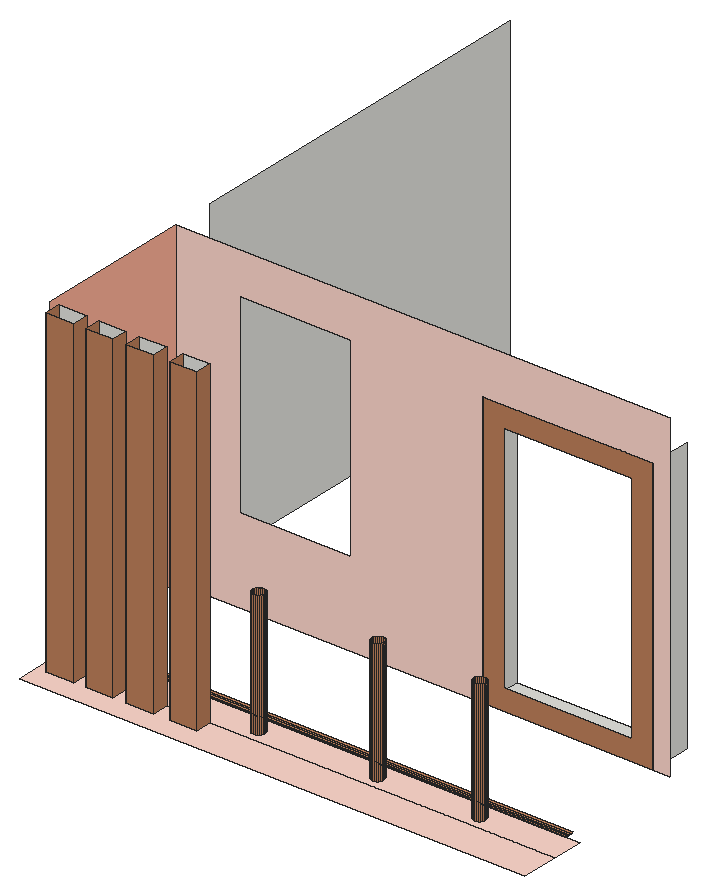
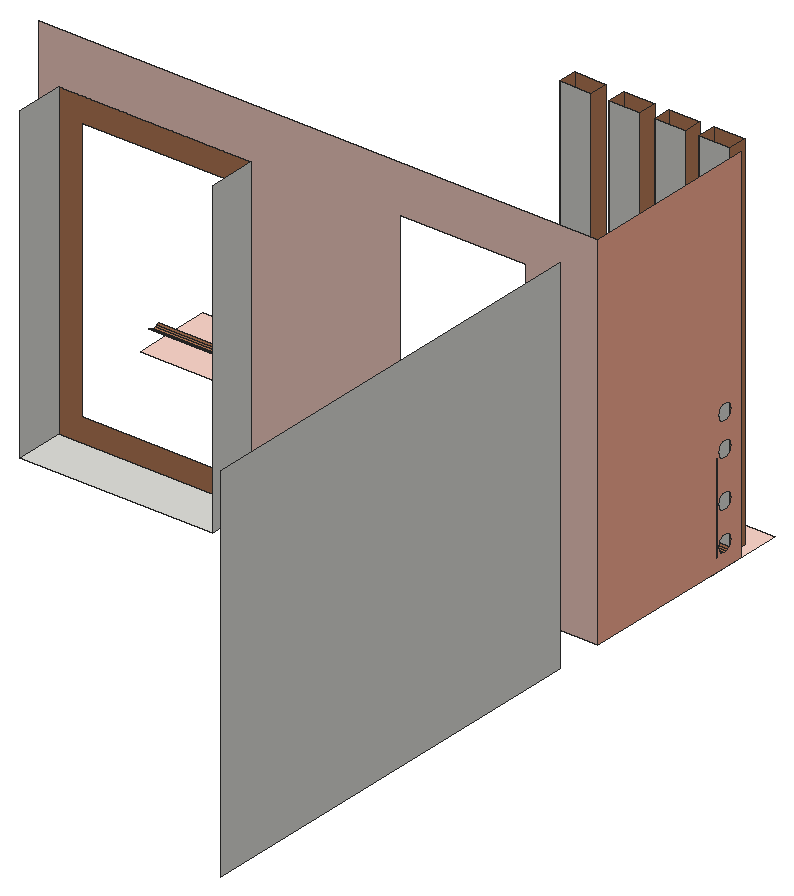
# SketchUp Ruby script. Lengths in inches.
U = 1.inch
M = Sketchup.active_model
def pt(a) = Geom::Point3d.new(a.map { |v| v * U })
def face(e, loops, mat)
  f = e.add_face(loops[0].map { |a| pt(a) })
  loops[1..].each { |l| e.add_face(l.map { |a| pt(a) }).erase! }
  f.material = f.back_material = mat if mat
  f
end
# faces: each face lists its corners as indices into pts; further lists are holes
def faces(e, pts, list, mat = nil) = list.each { |f| face(e, (f[0].is_a?(Array) ? f : [f]).map { |l| l.map { |i| pts[i] } }, mat) }
# xy, xz, yz: faces in a plane at the given z, y or x. An outline is a flat list of corners, or four numbers for a rectangle; further outlines are holes
def ring(l) = l.size == 4 ? [[l[0], l[1]], [l[2], l[1]], [l[2], l[3]], [l[0], l[3]]] : l.each_slice(2).to_a
def flat(e, list, mat, &to3) = list.each { |f| face(e, (f[0].is_a?(Array) ? f : [f]).map { |l| ring(l).map { |u, v| to3.(u, v) } }, mat) }
def xy(e, z, list, mat = nil) = flat(e, list, mat) { |x, y| [x, y, z] }
def xz(e, y, list, mat = nil) = flat(e, list, mat) { |x, z| [x, y, z] }
def yz(e, x, list, mat = nil) = flat(e, list, mat) { |y, z| [x, y, z] }
def lines(e, pts, list) = list.each { |a, b| e.add_line(pt(pts[a]), pt(pts[b])) }
# prism: a flat outline (further loops are holes) pulled along v
def prism(e, loops, v, mat = nil)
  f = face(e, loops, mat); d = Geom::Vector3d.new(v.map { |x| x * U })
  f.pushpull(f.normal.samedirection?(d) ? d.length : -d.length)
end
def box(e, o, s, mat = nil) = prism(e, [[o, [o[0] + s[0], o[1], o[2]], [o[0] + s[0], o[1] + s[1], o[2]], [o[0], o[1] + s[1], o[2]]]], [0, 0, s[2]], mat)
def at(x, y, z, deg = 0) = Geom::Transformation.translation(pt([x, y, z])) * Geom::Transformation.rotation(ORIGIN, Z_AXIS, deg.degrees)
def axes(o, x, y, z) = Geom::Transformation.new([*x, 0, *y, 0, *z, 0, *pt(o).to_a, 1])
def part(name) = M.definitions.add(name)
# library, detail: a bought-in or finely detailed component or shape, given as its bounding box
def library(name, o, s) = part(name).tap { |d| box(d.entities, o, s) }
def detail(e, o, s) = box(e.add_group.entities, o, s)
def put(e, d, t, mat = nil) = e.add_instance(d, t).tap { |i| i.material = mat if mat }
def group(e, t, mat = nil) = e.add_group.tap { |g| g.transformation = t; g.material = mat if mat }.entities
root = M.entities
M.materials.add("[Color B01]").color = [255, 216, 204]
M.materials.add("[Color B02]").color = [255, 178, 153]
M.materials.add("[Wood Veneer 02]").color = [190, 128, 91]
xy(root,700.1875,[[111.625,281.88,108.53,282.28,105.66,283.48,103.18,285.375,101.29,287.85,100.09,290.73,99.6875,293.82,100.09,296.91,101.29,299.78,103.18,302.26,105.66,304.15,108.53,305.35,111.625,305.75,114.71,305.35,117.59,304.15,120.06,302.26,121.96,299.78,123.15,296.91,123.5625,293.82,123.15,290.73,121.96,287.85,120.06,285.375,117.59,283.48,114.71,282.28],[267.125,281.88,264.03,282.28,261.16,283.48,258.68,285.375,256.79,287.85,255.59,290.73,255.1875,293.82,255.59,296.91,256.79,299.78,258.68,302.26,261.16,304.15,264.03,305.35,267.125,305.75,270.21,305.35,273.09,304.15,275.56,302.26,277.46,299.78,278.65,296.91,279.0625,293.82,278.65,290.73,277.46,287.85,275.56,285.375,273.09,283.48,270.21,282.28],[459.6875,281.88,456.6,282.28,453.72,283.48,451.25,285.375,449.35,287.85,448.16,290.73,447.75,293.82,448.16,296.91,449.35,299.78,451.25,302.26,453.72,304.15,456.6,305.35,459.6875,305.75,462.78,305.35,465.66,304.15,468.13,302.26,470.02,299.78,471.22,296.91,471.625,293.82,471.22,290.73,470.02,287.85,468.13,285.375,465.66,283.48,462.78,282.28],[690.375,281.88,687.28,282.28,684.41,283.48,681.93,285.375,680.04,287.85,678.84,290.73,678.4375,293.82,678.84,296.91,680.04,299.78,681.93,302.26,684.41,304.15,687.28,305.35,690.375,305.75,693.46,305.35,696.34,304.15,698.81,302.26,700.71,299.78,701.9,296.91,702.3125,293.82,701.9,290.73,700.71,287.85,698.81,285.375,696.34,283.48,693.46,282.28],[887.4375,281.88,884.35,282.28,881.47,283.48,879,285.375,877.1,287.85,875.91,290.73,875.5,293.82,875.91,296.91,877.1,299.78,879,302.26,881.47,304.15,884.35,305.35,887.4375,305.75,890.53,305.35,893.41,304.15,895.88,302.26,897.77,299.78,898.97,296.91,899.375,293.82,898.97,290.73,897.77,287.85,895.88,285.375,893.41,283.48,890.53,282.28],
  [670.44,571.9,998.42,653.97]])
xy(root,700.1875,[[77.93,195.0625,1053.15,195.0625,1053.15,267.5625,386.37,267.5625,386.37,236.1875,333.31,236.1875,333.31,267.5625,302.56,267.5625,302.56,236.1875,249.5,236.1875,249.5,267.5625,224.5,267.5625,224.5,236.1875,171.43,236.1875,171.43,267.5625,148.18,267.5625,148.18,236.1875,95.12,236.1875,95.12,267.5625,77.93,267.5625],[[77.93,267.5625,1053.15,328.8],[111.625,281.88,108.53,282.28,105.66,283.48,103.18,285.375,101.29,287.85,100.09,290.73,99.6875,293.82,100.09,296.91,101.29,299.78,103.18,302.26,105.66,304.15,108.53,305.35,111.625,305.75,114.71,305.35,117.59,304.15,120.06,302.26,121.96,299.78,123.15,296.91,123.5625,293.82,123.15,290.73,121.96,287.85,120.06,285.375,117.59,283.48,114.71,282.28],[887.4375,281.88,884.35,282.28,881.47,283.48,879,285.375,877.1,287.85,875.91,290.73,875.5,293.82,875.91,296.91,877.1,299.78,879,302.26,881.47,304.15,884.35,305.35,887.4375,305.75,890.53,305.35,893.41,304.15,895.88,302.26,897.77,299.78,898.97,296.91,899.375,293.82,898.97,290.73,897.77,287.85,895.88,285.375,893.41,283.48,890.53,282.28],[267.125,281.88,264.03,282.28,261.16,283.48,258.68,285.375,256.79,287.85,255.59,290.73,255.1875,293.82,255.59,296.91,256.79,299.78,258.68,302.26,261.16,304.15,264.03,305.35,267.125,305.75,270.21,305.35,273.09,304.15,275.56,302.26,277.46,299.78,278.65,296.91,279.0625,293.82,278.65,290.73,277.46,287.85,275.56,285.375,273.09,283.48,270.21,282.28],[690.375,281.88,687.28,282.28,684.41,283.48,681.93,285.375,680.04,287.85,678.84,290.73,678.4375,293.82,678.84,296.91,680.04,299.78,681.93,302.26,684.41,304.15,687.28,305.35,690.375,305.75,693.46,305.35,696.34,304.15,698.81,302.26,700.71,299.78,701.9,296.91,702.3125,293.82,701.9,290.73,700.71,287.85,698.81,285.375,696.34,283.48,693.46,282.28],[459.6875,281.88,456.6,282.28,453.72,283.48,451.25,285.375,449.35,287.85,448.16,290.73,447.75,293.82,448.16,296.91,449.35,299.78,451.25,302.26,453.72,304.15,456.6,305.35,459.6875,305.75,462.78,305.35,465.66,304.15,468.13,302.26,470.02,299.78,471.22,296.91,471.625,293.82,471.22,290.73,470.02,287.85,468.13,285.375,465.66,283.48,462.78,282.28]]],"[Color B01]")
xz(root,236.1875,[[95.12,700.1875,148.18,1321.0625],[171.43,700.1875,224.5,1321.0625],[249.5,700.1875,302.56,1321.0625],[333.31,700.1875,386.37,1321.0625]],"[Wood Veneer 02]")
xz(root,267.5625,[[95.12,700.1875,148.18,1321.0625],[171.43,700.1875,224.5,1321.0625],[249.5,700.1875,302.56,1321.0625],[333.31,700.1875,386.37,1321.0625]])
xz(root,571.9,[[[77.93,700.1875,670.44,700.1875,670.44,1230.86,998.42,1230.86,998.42,700.1875,1031.89,700.1875,1031.89,1321.0625,77.93,1321.0625],[200.6,864.76,415.54,1240.57]]],"[Color B01]")
xz(root,571.9,[[[670.44,700.1875,998.42,1230.86],[710.6,740.34,958.26,1190.71]]],"[Wood Veneer 02]")
yz(root,77.93,[[653.97,700.1875,1377.24,1321.0625]])
yz(root,77.93,[[[267.5625,700.1875,571.9,1321.0625],[300.66,924.24,297,924.72,293.6,926.13,290.67,928.38,288.43,931.3,287.02,934.71,286.54,938.37,287.02,942.02,288.43,945.43,290.67,948.35,293.6,950.6,297,952.01,300.66,952.49,304.32,952.01,307.72,950.6,310.65,948.35,312.89,945.43,314.3,942.02,314.79,938.37,314.3,934.71,312.89,931.3,310.65,928.38,307.72,926.13,304.32,924.72],[300.66,867.43,297,867.91,293.6,869.32,290.67,871.57,288.43,874.49,287.02,877.9,286.54,881.55,287.02,885.21,288.43,888.62,290.67,891.54,293.6,893.79,297,895.2,300.66,895.68,304.32,895.2,307.72,893.79,310.65,891.54,312.89,888.62,314.3,885.21,314.79,881.55,314.3,877.9,312.89,874.49,310.65,871.57,307.72,869.32,304.32,867.91],[300.66,787.68,297,788.16,293.6,789.57,290.67,791.82,288.43,794.74,287.02,798.15,286.54,801.8,287.02,805.46,288.43,808.87,290.67,811.79,293.6,814.04,297,815.45,300.66,815.93,304.32,815.45,307.72,814.04,310.65,811.79,312.89,808.87,314.3,805.46,314.79,801.8,314.3,798.15,312.89,794.74,310.65,791.82,307.72,789.57,304.32,788.16],[300.66,723.18,297,723.66,293.6,725.07,290.67,727.32,288.43,730.24,287.02,733.65,286.54,737.3,287.02,740.96,288.43,744.37,290.67,747.29,293.6,749.54,297,750.95,300.66,751.43,304.32,750.95,307.72,749.54,310.65,747.29,312.89,744.37,314.3,740.96,314.79,737.3,314.3,733.65,312.89,730.24,310.65,727.32,307.72,725.07,304.32,723.66]]],"[Color B02]")
yz(root,95.12,[[236.1875,700.1875,267.5625,1321.0625]],"[Wood Veneer 02]")
yz(root,148.18,[[236.1875,700.1875,267.5625,1321.0625]],"[Wood Veneer 02]")
yz(root,171.43,[[236.1875,700.1875,267.5625,1321.0625]],"[Wood Veneer 02]")
yz(root,224.5,[[236.1875,700.1875,267.5625,1321.0625]],"[Wood Veneer 02]")
yz(root,249.5,[[236.1875,700.1875,267.5625,1321.0625]],"[Wood Veneer 02]")
yz(root,302.56,[[236.1875,700.1875,267.5625,1321.0625]],"[Wood Veneer 02]")
yz(root,333.31,[[236.1875,700.1875,267.5625,1321.0625]],"[Wood Veneer 02]")
yz(root,386.37,[[236.1875,700.1875,267.5625,1321.0625]],"[Wood Veneer 02]")
yz(root,670.44,[[571.9,700.1875,653.97,1230.86]])
yz(root,998.42,[[571.9,700.1875,653.97,1230.86]])
p = [[108.53,282.28,700.1875],[111.625,281.88,700.1875],[111.625,281.88,945.43],[108.53,282.28,945.43],[114.71,282.28,700.1875],[114.71,282.28,945.43],
  [264.03,282.28,700.1875],[267.125,281.88,700.1875],[267.125,281.88,939.75],[264.03,282.28,939.75],[270.21,282.28,700.1875],[270.21,282.28,939.75],
  [456.6,282.28,700.1875],[459.6875,281.88,700.1875],[459.6875,281.88,941.3125],[456.6,282.28,941.3125],[462.78,282.28,700.1875],[462.78,282.28,941.3125],
  [687.28,282.28,700.1875],[690.375,281.88,700.1875],[690.375,281.88,938.37],[687.28,282.28,938.37],[693.46,282.28,700.1875],[693.46,282.28,938.37],
  [884.35,282.28,700.1875],[887.4375,281.88,700.1875],[887.4375,281.88,937.9375],[884.35,282.28,937.9375],[890.53,282.28,700.1875],[890.53,282.28,937.9375],
  [105.66,283.48,700.1875],[105.66,283.48,945.43],[117.59,283.48,700.1875],[117.59,283.48,945.43],[261.16,283.48,700.1875],[261.16,283.48,939.75],
  [273.09,283.48,700.1875],[273.09,283.48,939.75],[453.72,283.48,700.1875],[453.72,283.48,941.3125],[465.66,283.48,700.1875],[465.66,283.48,941.3125],
  [684.41,283.48,700.1875],[684.41,283.48,938.37],[696.34,283.48,700.1875],[696.34,283.48,938.37],[881.47,283.48,700.1875],[881.47,283.48,937.9375],
  [893.41,283.48,700.1875],[893.41,283.48,937.9375],[103.18,285.375,700.1875],[103.18,285.375,945.43],[120.06,285.375,700.1875],[120.06,285.375,945.43],
  [258.68,285.375,700.1875],[258.68,285.375,939.75],[275.56,285.375,700.1875],[275.56,285.375,939.75],[451.25,285.375,700.1875],[451.25,285.375,941.3125],
  [468.13,285.375,700.1875],[468.13,285.375,941.3125],[681.93,285.375,700.1875],[681.93,285.375,938.37],[698.81,285.375,700.1875],[698.81,285.375,938.37],
  [879,285.375,700.1875],[879,285.375,937.9375],[895.88,285.375,700.1875],[895.88,285.375,937.9375],[101.29,287.85,700.1875],[101.29,287.85,945.43],
  [121.96,287.85,700.1875],[121.96,287.85,945.43],[256.79,287.85,700.1875],[256.79,287.85,939.75],[277.46,287.85,700.1875],[277.46,287.85,939.75],
  [449.35,287.85,700.1875],[449.35,287.85,941.3125],[470.02,287.85,700.1875],[470.02,287.85,941.3125],[680.04,287.85,700.1875],[681.04,286.54,938.37],
  [680.04,287.85,938.37],[700.71,287.85,700.1875],[700.71,287.85,938.37],[699.71,286.54,938.37],[877.1,287.85,700.1875],[877.1,287.85,937.9375],
  [897.77,287.85,700.1875],[897.77,287.85,937.9375],[100.09,290.73,700.1875],[101.05,288.43,945.43],[100.09,290.73,945.43],[123.15,290.73,700.1875],
  [123.15,290.73,945.43],[122.2,288.43,945.43],[255.59,290.73,700.1875],[255.59,290.73,939.75],[278.65,290.73,700.1875],[278.65,290.73,939.75],
  [448.16,290.73,700.1875],[448.16,290.73,941.3125],[471.22,290.73,700.1875],[471.22,290.73,941.3125],[678.84,290.73,700.1875],[678.84,290.73,938.37],
  [701.9,290.73,700.1875],[701.9,290.73,938.37],[875.91,290.73,700.1875],[875.91,290.73,937.9375],[898.97,290.73,700.1875],[898.97,290.73,937.9375],
  [99.6875,293.82,700.1875],[99.6875,293.82,945.43],[123.5625,293.82,700.1875],[123.5625,293.82,945.43],[255.1875,293.82,700.1875],[255.1875,293.82,939.75],
  [279.0625,293.82,700.1875],[279.0625,293.82,939.75],[447.75,293.82,700.1875],[447.75,293.82,941.3125],[471.625,293.82,700.1875],[471.625,293.82,941.3125],
  [678.4375,293.82,700.1875],[678.4375,293.82,938.37],[702.3125,293.82,700.1875],[702.3125,293.82,938.37],[875.5,293.82,700.1875],[875.5,293.82,937.9375],
  [899.375,293.82,700.1875],[899.375,293.82,937.9375],[100.09,296.91,700.1875],[100.09,296.91,945.43],[123.15,296.91,700.1875],[123.15,296.91,945.43],
  [255.59,296.91,700.1875],[255.59,296.91,939.75],[278.65,296.91,700.1875],[278.65,296.91,939.75],[448.16,296.91,700.1875],[448.16,296.91,941.3125],
  [471.22,296.91,700.1875],[471.22,296.91,941.3125],[678.84,296.91,700.1875],[678.84,296.91,938.37],[701.9,296.91,700.1875],[701.9,296.91,938.37],
  [875.91,296.91,700.1875],[875.91,296.91,937.9375],[898.97,296.91,700.1875],[898.97,296.91,937.9375],[101.29,299.78,700.1875],[101.29,299.78,945.43],
  [121.96,299.78,700.1875],[121.96,299.78,945.43],[256.79,299.78,700.1875],[256.79,299.78,939.75],[277.46,299.78,700.1875],[277.46,299.78,939.75],
  [449.35,299.78,700.1875],[449.35,299.78,941.3125],[470.02,299.78,700.1875],[470.02,299.78,941.3125],[680.04,299.78,700.1875],[680.04,299.78,938.37],
  [700.71,299.78,700.1875],[700.71,299.78,938.37],[877.1,299.78,700.1875],[877.1,299.78,937.9375],[897.77,299.78,700.1875],[897.77,299.78,937.9375],
  [103.18,302.26,700.1875],[103.18,302.26,945.43],[120.06,302.26,700.1875],[120.06,302.26,945.43],[258.68,302.26,700.1875],[258.68,302.26,939.75],
  [275.56,302.26,700.1875],[275.56,302.26,939.75],[451.25,302.26,700.1875],[451.25,302.26,941.3125],[468.13,302.26,700.1875],[468.13,302.26,941.3125],
  [681.93,302.26,700.1875],[681.93,302.26,938.37],[698.81,302.26,700.1875],[698.81,302.26,938.37],[879,302.26,700.1875],[879,302.26,937.9375],
  [895.88,302.26,700.1875],[895.88,302.26,937.9375],[105.66,304.15,700.1875],[105.66,304.15,945.43],[117.59,304.15,700.1875],[117.59,304.15,945.43],
  [261.16,304.15,700.1875],[261.16,304.15,939.75],[273.09,304.15,700.1875],[273.09,304.15,939.75],[453.72,304.15,700.1875],[453.72,304.15,941.3125],
  [465.66,304.15,700.1875],[465.66,304.15,941.3125],[684.41,304.15,700.1875],[684.41,304.15,938.37],[696.34,304.15,700.1875],[696.34,304.15,938.37],
  [881.47,304.15,700.1875],[881.47,304.15,937.9375],[893.41,304.15,700.1875],[893.41,304.15,937.9375],[108.53,305.35,700.1875],[108.53,305.35,945.43],
  [114.71,305.35,700.1875],[114.71,305.35,945.43],[264.03,305.35,700.1875],[264.03,305.35,939.75],[270.21,305.35,700.1875],[270.21,305.35,939.75],
  [456.6,305.35,700.1875],[456.6,305.35,941.3125],[462.78,305.35,700.1875],[462.78,305.35,941.3125],[687.28,305.35,700.1875],[687.28,305.35,938.37],
  [693.46,305.35,700.1875],[693.46,305.35,938.37],[884.35,305.35,700.1875],[884.35,305.35,937.9375],[890.53,305.35,700.1875],[890.53,305.35,937.9375],
  [111.625,305.75,700.1875],[111.625,305.75,945.43],[267.125,305.75,700.1875],[267.125,305.75,939.75],[459.6875,305.75,700.1875],[459.6875,305.75,941.3125],
  [690.375,305.75,700.1875],[690.375,305.75,938.37],[887.4375,305.75,700.1875],[887.4375,305.75,937.9375],[1053.15,300.66,723.18],[1053.15,297,723.66],
  [77.93,297,723.66],[77.93,300.66,723.18],[1053.15,304.32,723.66],[77.93,304.32,723.66],[1053.15,293.6,725.07],[77.93,293.6,725.07],
  [1053.15,307.72,725.07],[77.93,307.72,725.07],[1053.15,290.67,727.32],[77.93,290.67,727.32],[1053.15,310.65,727.32],[77.93,310.65,727.32]]
faces(root,p,[[0,1,2,3],[1,4,5,2],[6,7,8,9],[7,10,11,8],[12,13,14,15],[13,16,17,14],[18,19,20,21],[19,22,23,20],
  [24,25,26,27],[25,28,29,26],[30,0,3,31],[4,32,33,5],[34,6,9,35],[10,36,37,11],[38,12,15,39],[16,40,41,17],
  [42,18,21,43],[22,44,45,23],[46,24,27,47],[28,48,49,29],[50,30,31,51],[32,52,53,33],[54,34,35,55],[36,56,57,37],
  [58,38,39,59],[40,60,61,41],[62,42,43,63],[44,64,65,45],[66,46,47,67],[48,68,69,49],[70,50,51,71],[52,72,73,53],
  [74,54,55,75],[56,76,77,57],[78,58,59,79],[60,80,81,61],[82,62,63,83,84],[64,85,86,87,65],[88,66,67,89],[68,90,91,69],
  [92,70,71,93,94],[72,95,96,97,73],[98,74,75,99],[76,100,101,77],[102,78,79,103],[80,104,105,81],[106,82,84,107],[85,108,109,86],
  [110,88,89,111],[90,112,113,91],[114,92,94,115],[95,116,117,96],[118,98,99,119],[100,120,121,101],[122,102,103,123],[104,124,125,105],
  [126,106,107,127],[108,128,129,109],[130,110,111,131],[112,132,133,113],[134,114,115,135],[116,136,137,117],[138,118,119,139],[120,140,141,121],
  [142,122,123,143],[124,144,145,125],[146,126,127,147],[128,148,149,129],[150,130,131,151],[132,152,153,133],[154,134,135,155],[136,156,157,137],
  [158,138,139,159],[140,160,161,141],[162,142,143,163],[144,164,165,145],[166,146,147,167],[148,168,169,149],[170,150,151,171],[152,172,173,153],
  [174,154,155,175],[156,176,177,157],[178,158,159,179],[160,180,181,161],[182,162,163,183],[164,184,185,165],[186,166,167,187],[168,188,189,169],
  [190,170,171,191],[172,192,193,173],[194,174,175,195],[176,196,197,177],[198,178,179,199],[180,200,201,181],[202,182,183,203],[184,204,205,185],
  [206,186,187,207],[188,208,209,189],[210,190,191,211],[192,212,213,193],[214,194,195,215],[196,216,217,197],[218,198,199,219],[200,220,221,201],
  [222,202,203,223],[204,224,225,205],[226,206,207,227],[208,228,229,209],[230,210,211,231],[212,232,233,213],[234,214,215,235],[216,234,235,217],
  [236,218,219,237],[220,236,237,221],[238,222,223,239],[224,238,239,225],[240,226,227,241],[228,240,241,229],[242,230,231,243],[232,242,243,233],
  [244,245,246,247],[248,244,247,249],[245,250,251,246],[252,248,249,253],[250,254,255,251],[256,252,253,257]],"[Wood Veneer 02]")
